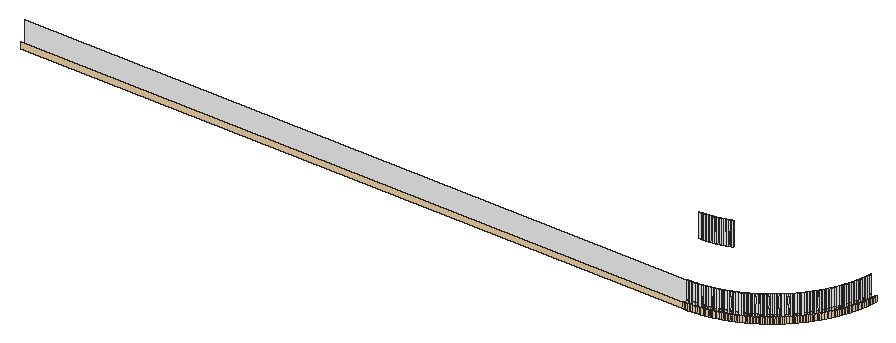
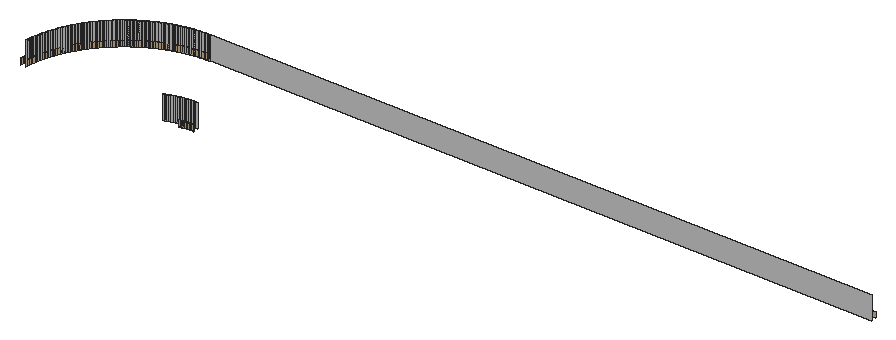
# SketchUp Ruby script. Lengths in inches.
U = 1.inch
M = Sketchup.active_model
def pt(a) = Geom::Point3d.new(a.map { |v| v * U })
def face(e, loops, mat)
  f = e.add_face(loops[0].map { |a| pt(a) })
  loops[1..].each { |l| e.add_face(l.map { |a| pt(a) }).erase! }
  f.material = f.back_material = mat if mat
  f
end
# faces: each face lists its corners as indices into pts; further lists are holes
def faces(e, pts, list, mat = nil) = list.each { |f| face(e, (f[0].is_a?(Array) ? f : [f]).map { |l| l.map { |i| pts[i] } }, mat) }
# xy, xz, yz: faces in a plane at the given z, y or x. An outline is a flat list of corners, or four numbers for a rectangle; further outlines are holes
def ring(l) = l.size == 4 ? [[l[0], l[1]], [l[2], l[1]], [l[2], l[3]], [l[0], l[3]]] : l.each_slice(2).to_a
def flat(e, list, mat, &to3) = list.each { |f| face(e, (f[0].is_a?(Array) ? f : [f]).map { |l| ring(l).map { |u, v| to3.(u, v) } }, mat) }
def xy(e, z, list, mat = nil) = flat(e, list, mat) { |x, y| [x, y, z] }
def xz(e, y, list, mat = nil) = flat(e, list, mat) { |x, z| [x, y, z] }
def yz(e, x, list, mat = nil) = flat(e, list, mat) { |y, z| [x, y, z] }
def lines(e, pts, list) = list.each { |a, b| e.add_line(pt(pts[a]), pt(pts[b])) }
# prism: a flat outline (further loops are holes) pulled along v
def prism(e, loops, v, mat = nil)
  f = face(e, loops, mat); d = Geom::Vector3d.new(v.map { |x| x * U })
  f.pushpull(f.normal.samedirection?(d) ? d.length : -d.length)
end
def box(e, o, s, mat = nil) = prism(e, [[o, [o[0] + s[0], o[1], o[2]], [o[0] + s[0], o[1] + s[1], o[2]], [o[0], o[1] + s[1], o[2]]]], [0, 0, s[2]], mat)
def at(x, y, z, deg = 0) = Geom::Transformation.translation(pt([x, y, z])) * Geom::Transformation.rotation(ORIGIN, Z_AXIS, deg.degrees)
def axes(o, x, y, z) = Geom::Transformation.new([*x, 0, *y, 0, *z, 0, *pt(o).to_a, 1])
def part(name) = M.definitions.add(name)
# library, detail: a bought-in or finely detailed component or shape, given as its bounding box
def library(name, o, s) = part(name).tap { |d| box(d.entities, o, s) }
def detail(e, o, s) = box(e.add_group.entities, o, s)
def put(e, d, t, mat = nil) = e.add_instance(d, t).tap { |i| i.material = mat if mat }
def group(e, t, mat = nil) = e.add_group.tap { |g| g.transformation = t; g.material = mat if mat }.entities
root = M.entities
M.materials.add("False Ceiling Light").color = [254, 223, 179]
M.materials.add("[Quartz Light Grey]").color = [251, 251, 252]
xz(root,43.5,[[45,115.32,177,116.49],[177,115.32,177.24,116.49],[177.24,115.32,177.47,116.49]],"False Ceiling Light")
xz(root,44.5,[[176.99,115.32,177.23,116.49],[177.23,115.32,177.45,116.49]],"False Ceiling Light")
xz(root,44.5,[[45.01,115.32,176.99,120],[176.99,115.32,177.23,120],[177.23,115.32,177.45,120]],"[Quartz Light Grey]")
xz(root,62.5,[[165.01,115.32,165.2,120]],"[Quartz Light Grey]")
xz(root,62.51,[[165.41,115.32,165.61,120]],"[Quartz Light Grey]")
xz(root,63.5,[[165.01,115.32,165.19,116.49],[165.19,115.32,165.38,116.49]],"False Ceiling Light")
p = [[177.47,43.5,115.32],[177.71,43.51,115.32],[177.71,43.51,116.49],[177.47,43.5,116.49],[177.94,43.52,115.32],[177.94,43.52,116.49],
  [178.18,43.53,115.32],[178.18,43.53,116.49],[178.41,43.54,115.32],[178.41,43.54,116.49],[178.65,43.56,115.32],[178.65,43.56,116.49],
  [178.88,43.58,115.32],[178.88,43.58,116.49],[179.12,43.6,115.32],[179.12,43.6,116.49],[179.35,43.625,115.32],[179.35,43.625,116.49],
  [179.59,43.65,115.32],[179.59,43.65,116.49],[179.82,43.68,115.32],[179.82,43.68,116.49],[180.05,43.71,115.32],[180.05,43.71,116.49],
  [180.29,43.74,115.32],[180.29,43.74,116.49],[180.52,43.78,115.32],[180.52,43.78,116.49],[180.75,43.82,115.32],[180.75,43.82,116.49],
  [180.98,43.86,115.32],[180.98,43.86,116.49],[181.22,43.9,115.32],[181.22,43.9,116.49],[181.45,43.94,115.32],[181.45,43.94,116.49],
  [181.68,43.99,115.32],[181.68,43.99,116.49],[181.91,44.04,115.32],[181.91,44.04,116.49],[182.14,44.09,115.32],[182.14,44.09,116.49],
  [182.37,44.15,115.32],[182.37,44.15,116.49],[182.6,44.21,115.32],[182.6,44.21,116.49],[182.82,44.27,115.32],[182.82,44.27,116.49],
  [183.05,44.33,115.32],[183.05,44.33,116.49],[183.28,44.39,115.32],[183.28,44.39,116.49],[183.5,44.46,115.32],[183.5,44.46,116.49],
  [177.45,44.5,115.32],[177.68,44.51,115.32],[177.68,44.51,120],[177.45,44.5,120],[177.68,44.51,115.32],[177.45,44.5,115.32],
  [177.45,44.5,116.49],[177.68,44.51,116.49],[177.9,44.52,115.32],[177.9,44.52,120],[177.9,44.52,115.32],[177.9,44.52,116.49],
  [178.125,44.53,115.32],[178.125,44.53,120],[178.125,44.53,115.32],[178.125,44.53,116.49],[178.35,44.54,115.32],[178.35,44.54,120],
  [178.35,44.54,115.32],[178.35,44.54,116.49],[178.57,44.56,115.32],[178.57,44.56,120],[178.57,44.56,115.32],[178.57,44.56,116.49],
  [183.73,44.53,115.32],[183.73,44.53,116.49],[183.95,44.6,115.32],[183.95,44.6,116.49],[178.8,44.58,115.32],[178.8,44.58,120],
  [178.8,44.58,115.32],[178.8,44.58,116.49],[179.02,44.6,115.32],[179.02,44.6,120],[179.02,44.6,115.32],[179.02,44.6,116.49],
  [179.25,44.62,115.32],[179.25,44.62,120],[179.25,44.62,115.32],[179.25,44.62,116.49],[179.47,44.64,115.32],[179.47,44.64,120],
  [179.47,44.64,115.32],[179.47,44.64,116.49],[179.69,44.67,115.32],[179.69,44.67,120],[179.69,44.67,115.32],[179.69,44.67,116.49],
  [184.18,44.68,115.32],[184.18,44.68,116.49],[179.92,44.7,115.32],[179.92,44.7,120],[179.92,44.7,115.32],[179.92,44.7,116.49],
  [180.14,44.73,115.32],[180.14,44.73,120],[180.14,44.73,115.32],[180.14,44.73,116.49],[180.36,44.76,115.32],[180.36,44.76,120],
  [180.36,44.76,115.32],[180.36,44.76,116.49],[184.4,44.75,115.32],[184.4,44.75,116.49],[180.59,44.8,115.32],[180.59,44.8,120],
  [180.59,44.8,115.32],[180.59,44.8,116.49],[180.81,44.84,115.32],[180.81,44.84,120],[180.81,44.84,115.32],[180.81,44.84,116.49],
  [181.03,44.88,115.32],[181.03,44.88,120],[181.03,44.88,115.32],[181.03,44.88,116.49],[184.62,44.83,115.32],[184.62,44.83,116.49],
  [184.84,44.91,115.32],[184.84,44.91,116.49],[181.25,44.92,115.32],[181.25,44.92,120],[181.25,44.92,115.32],[181.25,44.92,116.49],
  [181.47,44.97,115.32],[181.47,44.97,120],[181.47,44.97,115.32],[181.47,44.97,116.49],[185.0625,44.99,115.32],[185.0625,44.99,116.49],
  [181.69,45.02,115.32],[181.69,45.02,120],[181.69,45.02,115.32],[181.69,45.02,116.49],[181.91,45.07,115.32],[181.91,45.07,120],
  [181.91,45.07,115.32],[181.91,45.07,116.49],[185.28,45.08,115.32],[185.28,45.08,116.49],[182.13,45.12,115.32],[182.13,45.12,120],
  [182.13,45.12,115.32],[182.13,45.12,116.49],[182.35,45.18,115.32],[182.35,45.18,120],[182.35,45.18,115.32],[182.35,45.18,116.49],
  [185.5,45.17,115.32],[185.5,45.17,116.49],[182.56,45.23,115.32],[182.56,45.23,120],[182.56,45.23,115.32],[182.56,45.23,116.49],
  [182.78,45.29,115.32],[182.78,45.29,120],[182.78,45.29,115.32],[182.78,45.29,116.49],[185.72,45.26,115.32],[185.72,45.26,116.49],
  [183,45.35,115.32],[183,45.35,120],[183,45.35,115.32],[183,45.35,116.49],[185.9375,45.35,115.32],[185.9375,45.35,116.49],
  [183.21,45.42,115.32],[183.21,45.42,120],[183.21,45.42,115.32],[183.21,45.42,116.49],[183.43,45.48,115.32],[183.43,45.48,120],
  [183.43,45.48,115.32],[183.43,45.48,116.49],[186.15,45.45,115.32],[186.15,45.45,116.49],[186.37,45.54,115.32],[186.37,45.54,116.49],
  [183.64,45.55,115.32],[183.64,45.55,120],[183.64,45.55,115.32],[183.64,45.55,116.49],[186.58,45.64,115.32],[186.58,45.64,116.49],
  [183.86,45.625,115.32],[183.86,45.625,120],[183.86,45.625,115.32],[183.86,45.625,116.49],[184.07,45.7,115.32],[184.07,45.7,120],
  [184.07,45.7,115.32],[184.07,45.7,116.49],[186.79,45.74,115.32],[186.79,45.74,116.49],[184.28,45.77,115.32],[184.28,45.77,120],
  [184.28,45.77,115.32],[184.28,45.77,116.49],[187,45.85,115.32],[187,45.85,116.49],[184.49,45.85,115.32],[184.49,45.85,120],
  [184.49,45.85,115.32],[184.49,45.85,116.49],[184.7,45.93,115.32],[184.7,45.93,120],[184.7,45.93,115.32],[184.7,45.93,116.49],
  [187.21,45.95,115.32],[187.21,45.95,116.49],[184.91,46.01,115.32],[184.91,46.01,120],[184.91,46.01,115.32],[184.91,46.01,116.49],
  [185.125,46.09,115.32],[185.125,46.09,120],[185.125,46.09,115.32],[185.125,46.09,116.49],[187.42,46.06,115.32],[187.42,46.06,116.49],
  [185.33,46.18,115.32],[185.33,46.18,120],[185.33,46.18,115.32],[185.33,46.18,116.49],[187.63,46.17,115.32],[187.63,46.17,116.49],
  [185.54,46.27,115.32],[185.54,46.27,120],[185.54,46.27,115.32],[185.54,46.27,116.49],[187.84,46.28,115.32],[187.84,46.28,116.49],
  [185.74,46.36,115.32],[185.74,46.36,120],[185.74,46.36,115.32],[185.74,46.36,116.49],[188.05,46.4,115.32],[188.05,46.4,116.49],
  [185.95,46.45,115.32],[185.95,46.45,120],[185.95,46.45,115.32],[185.95,46.45,116.49],[188.25,46.51,115.32],[188.25,46.51,116.49],
  [186.15,46.55,115.32],[186.15,46.55,120],[186.15,46.55,115.32],[186.15,46.55,116.49],[186.36,46.64,115.32],[186.36,46.64,120],
  [186.36,46.64,115.32],[186.36,46.64,116.49],[188.45,46.63,115.32],[188.45,46.63,116.49],[186.56,46.74,115.32],[186.56,46.74,120],
  [186.56,46.74,115.32],[186.56,46.74,116.49],[188.66,46.75,115.32],[188.66,46.75,116.49],[186.76,46.84,115.32],[186.76,46.84,120],
  [186.76,46.84,115.32],[186.76,46.84,116.49],[186.96,46.95,115.32],[186.96,46.95,120],[186.96,46.95,115.32],[186.96,46.95,116.49],
  [188.86,46.88,115.32],[188.86,46.88,116.49],[187.16,47.05,115.32],[187.16,47.05,120],[187.16,47.05,115.32],[187.16,47.05,116.49],
  [189.06,47,115.32],[189.06,47,116.49],[189.25,47.13,115.32],[189.25,47.13,116.49],[187.36,47.16,115.32],[187.36,47.16,120],
  [187.36,47.16,115.32],[187.36,47.16,116.49],[189.45,47.26,115.32],[189.45,47.26,116.49],[187.55,47.27,115.32],[187.55,47.27,120],
  [187.55,47.27,115.32],[187.55,47.27,116.49],[187.75,47.38,115.32],[187.75,47.38,120],[187.75,47.38,115.32],[187.75,47.38,116.49],
  [189.65,47.39,115.32],[189.65,47.39,116.49],[187.94,47.49,115.32],[187.94,47.49,120],[187.94,47.49,115.32],[187.94,47.49,116.49],
  [189.84,47.52,115.32],[189.84,47.52,116.49],[188.14,47.61,115.32],[188.14,47.61,120],[188.14,47.61,115.32],[188.14,47.61,116.49],
  [190.03,47.66,115.32],[190.03,47.66,116.49],[188.33,47.73,115.32],[188.33,47.73,120],[188.33,47.73,115.32],[188.33,47.73,116.49],
  [188.52,47.85,115.32],[188.52,47.85,120],[188.52,47.85,115.32],[188.52,47.85,116.49],[190.23,47.8,115.32],[190.23,47.8,116.49],
  [188.71,47.97,115.32],[188.71,47.97,120],[188.71,47.97,115.32],[188.71,47.97,116.49],[190.42,47.9375,115.32],[190.42,47.9375,116.49],
  [190.6,48.08,115.32],[190.6,48.08,116.49],[188.9,48.09,115.32],[188.9,48.09,120],[188.9,48.09,115.32],[188.9,48.09,116.49],
  [189.08,48.22,115.32],[189.08,48.22,120],[189.08,48.22,115.32],[189.08,48.22,116.49],[190.79,48.22,115.32],[190.79,48.22,116.49],
  [189.27,48.35,115.32],[189.27,48.35,120],[189.27,48.35,115.32],[189.27,48.35,116.49],[190.98,48.37,115.32],[190.98,48.37,116.49],
  [189.45,48.47,115.32],[189.45,48.47,120],[189.45,48.47,115.32],[189.45,48.47,116.49],[191.16,48.51,115.32],[191.16,48.51,116.49],
  [189.64,48.61,115.32],[189.64,48.61,120],[189.64,48.61,115.32],[189.64,48.61,116.49],[191.34,48.66,115.32],[191.34,48.66,116.49],
  [189.82,48.74,115.32],[189.82,48.74,120],[189.82,48.74,115.32],[189.82,48.74,116.49],[190,48.875,115.32],[190,48.875,120],
  [190,48.875,115.32],[190,48.875,116.49],[191.52,48.81,115.32],[191.52,48.81,116.49],[191.7,48.97,115.32],[191.7,48.97,116.49],
  [190.18,49.01,115.32],[190.18,49.01,120],[190.18,49.01,115.32],[190.18,49.01,116.49],[190.35,49.15,115.32],[190.35,49.15,120],
  [190.35,49.15,115.32],[190.35,49.15,116.49],[191.88,49.12,115.32],[191.88,49.12,116.49],[192.06,49.28,115.32],[192.06,49.28,116.49],
  [190.53,49.29,115.32],[190.53,49.29,120],[190.53,49.29,115.32],[190.53,49.29,116.49],[190.7,49.43,115.32],[190.7,49.43,120],
  [190.7,49.43,115.32],[190.7,49.43,116.49],[192.23,49.4375,115.32],[192.23,49.4375,116.49],[190.88,49.58,115.32],[190.88,49.58,120],
  [190.88,49.58,115.32],[190.88,49.58,116.49],[192.4,49.6,115.32],[192.4,49.6,116.49],[191.05,49.72,115.32],[191.05,49.72,120],
  [191.05,49.72,115.32],[191.05,49.72,116.49],[192.57,49.76,115.32],[192.57,49.76,116.49],[191.22,49.87,115.32],[191.22,49.87,120],
  [191.22,49.87,115.32],[191.22,49.87,116.49],[192.74,49.92,115.32],[192.74,49.92,116.49],[191.39,50.02,115.32],[191.39,50.02,120],
  [191.39,50.02,115.32],[191.39,50.02,116.49],[192.91,50.09,115.32],[192.91,50.09,116.49],[191.55,50.17,115.32],[191.55,50.17,120],
  [191.55,50.17,115.32],[191.55,50.17,116.49],[193.08,50.26,115.32],[193.08,50.26,116.49],[191.72,50.33,115.32],[191.72,50.33,120],
  [191.72,50.33,115.32],[191.72,50.33,116.49],[191.88,50.48,115.32],[191.88,50.48,120],[191.88,50.48,115.32],[191.88,50.48,116.49],
  [193.24,50.43,115.32],[193.24,50.43,116.49],[193.4,50.6,115.32],[193.4,50.6,116.49],[192.04,50.64,115.32],[192.04,50.64,120],
  [192.04,50.64,115.32],[192.04,50.64,116.49],[192.2,50.8,115.32],[192.2,50.8,120],[192.2,50.8,115.32],[192.2,50.8,116.49],
  [193.5625,50.77,115.32],[193.5625,50.77,116.49],[192.36,50.96,115.32],[192.36,50.96,120],[192.36,50.96,115.32],[192.36,50.96,116.49],
  [193.72,50.94,115.32],[193.72,50.94,116.49],[193.88,51.12,115.32],[193.88,51.12,116.49],[192.52,51.12,115.32],[192.52,51.12,120],
  [192.52,51.12,115.32],[192.52,51.12,116.49],[192.67,51.28,115.32],[192.67,51.28,120],[192.67,51.28,115.32],[192.67,51.28,116.49],
  [194.03,51.3,115.32],[194.03,51.3,116.49],[192.83,51.45,115.32],[192.83,51.45,120],[192.83,51.45,115.32],[192.83,51.45,116.49],
  [194.19,51.48,115.32],[194.19,51.48,116.49],[192.98,51.61,115.32],[192.98,51.61,120],[192.98,51.61,115.32],[192.98,51.61,116.49],
  [194.34,51.66,115.32],[194.34,51.66,116.49],[193.13,51.78,115.32],[193.13,51.78,120],[193.13,51.78,115.32],[193.13,51.78,116.49],
  [194.49,51.84,115.32],[194.49,51.84,116.49],[193.28,51.95,115.32],[193.28,51.95,120],[193.28,51.95,115.32],[193.28,51.95,116.49],
  [194.63,52.02,115.32],[194.63,52.02,116.49],[193.42,52.12,115.32],[193.42,52.12,120],[193.42,52.12,115.32],[193.42,52.12,116.49],
  [194.78,52.21,115.32],[194.78,52.21,116.49],[193.57,52.3,115.32],[193.57,52.3,120],[193.57,52.3,115.32],[193.57,52.3,116.49],
  [194.92,52.4,115.32],[194.92,52.4,116.49],[193.71,52.47,115.32],[193.71,52.47,120],[193.71,52.47,115.32],[193.71,52.47,116.49],
  [195.0625,52.58,115.32],[195.0625,52.58,116.49],[193.85,52.65,115.32],[193.85,52.65,120],[193.85,52.65,115.32],[193.85,52.65,116.49],
  [193.99,52.82,115.32],[193.99,52.82,120],[193.99,52.82,115.32],[193.99,52.82,116.49],[195.2,52.77,115.32],[195.2,52.77,116.49],
  [194.125,53,115.32],[194.125,53,120],[194.125,53,115.32],[194.125,53,116.49],[195.34,52.97,115.32],[195.34,52.97,116.49],
  [194.26,53.18,115.32],[194.26,53.18,120],[194.26,53.18,115.32],[194.26,53.18,116.49],[195.48,53.16,115.32],[195.48,53.16,116.49],
  [194.39,53.36,115.32],[194.39,53.36,120],[194.39,53.36,115.32],[194.39,53.36,116.49],[195.61,53.35,115.32],[195.61,53.35,116.49],
  [194.53,53.55,115.32],[194.53,53.55,120],[194.53,53.55,115.32],[194.53,53.55,116.49],[195.74,53.55,115.32],[195.74,53.55,116.49],
  [194.65,53.73,115.32],[194.65,53.73,120],[194.65,53.73,115.32],[194.65,53.73,116.49],[195.87,53.75,115.32],[195.87,53.75,116.49],
  [194.78,53.92,115.32],[194.78,53.92,120],[194.78,53.92,115.32],[194.78,53.92,116.49],[196,53.94,115.32],[196,53.94,116.49],
  [194.91,54.1,115.32],[194.91,54.1,120],[194.91,54.1,115.32],[194.91,54.1,116.49],[196.12,54.14,115.32],[196.12,54.14,116.49],
  [195.03,54.29,115.32],[195.03,54.29,120],[195.03,54.29,115.32],[195.03,54.29,116.49],[196.25,54.34,115.32],[196.25,54.34,116.49],
  [195.15,54.48,115.32],[195.15,54.48,120],[195.15,54.48,115.32],[195.15,54.48,116.49],[196.37,54.55,115.32],[196.37,54.55,116.49],
  [195.27,54.67,115.32],[195.27,54.67,120],[195.27,54.67,115.32],[195.27,54.67,116.49],[196.49,54.75,115.32],[196.49,54.75,116.49],
  [195.39,54.86,115.32],[195.39,54.86,120],[195.39,54.86,115.32],[195.39,54.86,116.49],[196.6,54.95,115.32],[196.6,54.95,116.49],
  [195.51,55.06,115.32],[195.51,55.06,120],[195.51,55.06,115.32],[195.51,55.06,116.49],[196.72,55.16,115.32],[196.72,55.16,116.49],
  [195.62,55.25,115.32],[195.62,55.25,120],[195.62,55.25,115.32],[195.62,55.25,116.49],[196.83,55.37,115.32],[196.83,55.37,116.49],
  [195.73,55.45,115.32],[195.73,55.45,120],[195.73,55.45,115.32],[195.73,55.45,116.49],[195.84,55.64,115.32],[195.84,55.64,120],
  [195.84,55.64,115.32],[195.84,55.64,116.49],[196.94,55.58,115.32],[196.94,55.58,116.49],[195.95,55.84,115.32],[195.95,55.84,120],
  [195.95,55.84,115.32],[195.95,55.84,116.49],[197.05,55.79,115.32],[197.05,55.79,116.49],[196.05,56.04,115.32],[196.05,56.04,120],
  [196.05,56.04,115.32],[196.05,56.04,116.49],[197.15,56,115.32],[197.15,56,116.49],[196.16,56.24,115.32],[196.16,56.24,120],
  [196.16,56.24,115.32],[196.16,56.24,116.49],[197.26,56.21,115.32],[197.26,56.21,116.49],[196.26,56.44,115.32],[196.26,56.44,120],
  [196.26,56.44,115.32],[196.26,56.44,116.49],[197.36,56.42,115.32],[197.36,56.42,116.49],[196.36,56.64,115.32],[196.36,56.64,120],
  [196.36,56.64,115.32],[196.36,56.64,116.49],[197.46,56.63,115.32],[197.46,56.63,116.49],[196.45,56.85,115.32],[196.45,56.85,120],
  [196.45,56.85,115.32],[196.45,56.85,116.49],[197.55,56.85,115.32],[197.55,56.85,116.49],[196.55,57.05,115.32],[196.55,57.05,120],
  [196.55,57.05,115.32],[196.55,57.05,116.49],[197.65,57.0625,115.32],[197.65,57.0625,116.49],[196.64,57.26,115.32],[196.64,57.26,120],
  [196.64,57.26,115.32],[196.64,57.26,116.49],[197.74,57.28,115.32],[197.74,57.28,116.49],[196.73,57.46,115.32],[196.73,57.46,120],
  [196.73,57.46,115.32],[196.73,57.46,116.49],[197.83,57.5,115.32],[197.83,57.5,116.49],[196.82,57.67,115.32],[196.82,57.67,120],
  [196.82,57.67,115.32],[196.82,57.67,116.49],[197.92,57.72,115.32],[197.92,57.72,116.49],[196.91,57.875,115.32],[196.91,57.875,120],
  [196.91,57.875,115.32],[196.91,57.875,116.49],[198.01,57.9375,115.32],[198.01,57.9375,116.49],[196.99,58.09,115.32],[196.99,58.09,120],
  [196.99,58.09,115.32],[196.99,58.09,116.49],[198.09,58.16,115.32],[198.09,58.16,116.49],[197.07,58.3,115.32],[197.07,58.3,120],
  [197.07,58.3,115.32],[197.07,58.3,116.49],[198.17,58.38,115.32],[198.17,58.38,116.49],[197.15,58.51,115.32],[197.15,58.51,120],
  [197.15,58.51,115.32],[197.15,58.51,116.49],[198.25,58.6,115.32],[198.25,58.6,116.49],[197.23,58.72,115.32],[197.23,58.72,120],
  [197.23,58.72,115.32],[197.23,58.72,116.49],[198.32,58.82,115.32],[198.32,58.82,116.49],[197.3,58.93,115.32],[197.3,58.93,120],
  [197.3,58.93,115.32],[197.3,58.93,116.49],[198.4,59.05,115.32],[198.4,59.05,116.49],[197.375,59.14,115.32],[197.375,59.14,120],
  [197.375,59.14,115.32],[197.375,59.14,116.49],[198.47,59.27,115.32],[198.47,59.27,116.49],[197.45,59.36,115.32],[197.45,59.36,120],
  [197.45,59.36,115.32],[197.45,59.36,116.49],[198.54,59.5,115.32],[198.54,59.5,116.49],[197.52,59.57,115.32],[197.52,59.57,120],
  [197.52,59.57,115.32],[197.52,59.57,116.49],[198.61,59.72,115.32],[198.61,59.72,116.49],[197.58,59.79,115.32],[197.58,59.79,120],
  [197.58,59.79,115.32],[197.58,59.79,116.49],[198.67,59.95,115.32],[198.67,59.95,116.49],[197.65,60,115.32],[197.65,60,120],
  [197.65,60,115.32],[197.65,60,116.49],[198.73,60.18,115.32],[198.73,60.18,116.49],[197.71,60.22,115.32],[197.71,60.22,120],
  [197.71,60.22,115.32],[197.71,60.22,116.49],[197.77,60.44,115.32],[197.77,60.44,120],[197.77,60.44,115.32],[197.77,60.44,116.49],
  [198.79,60.4,115.32],[198.79,60.4,116.49],[197.82,60.65,115.32],[197.82,60.65,120],[197.82,60.65,115.32],[197.82,60.65,116.49],
  [198.85,60.63,115.32],[198.85,60.63,116.49],[198.91,60.86,115.32],[198.91,60.86,116.49],[197.88,60.87,115.32],[197.88,60.87,120],
  [197.88,60.87,115.32],[197.88,60.87,116.49],[197.93,61.09,115.32],[197.93,61.09,120],[197.93,61.09,115.32],[197.93,61.09,116.49],
  [198.96,61.09,115.32],[198.96,61.09,116.49],[197.98,61.31,115.32],[197.98,61.31,120],[197.98,61.31,115.32],[197.98,61.31,116.49],
  [199.01,61.32,115.32],[199.01,61.32,116.49],[198.03,61.53,115.32],[198.03,61.53,120],[198.03,61.53,115.32],[198.03,61.53,116.49],
  [199.06,61.55,115.32],[199.06,61.55,116.49],[198.08,61.75,115.32],[198.08,61.75,120],[198.08,61.75,115.32],[198.08,61.75,116.49],
  [199.1,61.78,115.32],[199.1,61.78,116.49],[198.12,61.97,115.32],[198.12,61.97,120],[198.12,61.97,115.32],[198.12,61.97,116.49],
  [199.14,62.02,115.32],[199.14,62.02,116.49],[198.16,62.19,115.32],[198.16,62.19,120],[198.16,62.19,115.32],[198.16,62.19,116.49],
  [199.18,62.25,115.32],[199.18,62.25,116.49],[198.2,62.41,115.32],[198.2,62.41,120],[198.2,62.41,115.32],[198.2,62.41,116.49],
  [199.22,62.48,115.32],[199.22,62.48,116.49],[198.24,62.64,115.32],[198.24,62.64,120],[198.24,62.64,115.32],[198.24,62.64,116.49],
  [165.41,62.51,115.32],[165.2,62.5,115.32],[165.2,62.5,120],[165.41,62.51,120],[165.8125,62.52,115.32],[165.61,62.51,115.32],
  [165.61,62.51,120],[165.8125,62.52,120],[166.01,62.53,115.32],[166.01,62.53,120],[166.22,62.55,115.32],[166.22,62.55,120],
  [166.42,62.56,115.32],[166.42,62.56,120],[199.26,62.71,115.32],[199.26,62.71,116.49],[166.62,62.58,115.32],[166.62,62.58,120],
  [166.82,62.61,115.32],[166.82,62.61,120],[167.02,62.63,115.32],[167.02,62.63,120],[167.22,62.66,115.32],[167.22,62.66,120],
  [198.27,62.86,115.32],[198.27,62.86,120],[198.27,62.86,115.32],[198.27,62.86,116.49],[167.42,62.69,115.32],[167.42,62.69,120],
  [167.625,62.72,115.32],[167.625,62.72,120],[167.82,62.76,115.32],[167.82,62.76,120],[199.29,62.95,115.32],[199.29,62.95,116.49],
  [168.02,62.8,115.32],[168.02,62.8,120],[168.22,62.84,115.32],[168.22,62.84,120],[168.42,62.88,115.32],[168.42,62.88,120],
  [168.62,62.93,115.32],[168.62,62.93,120],[168.82,62.98,115.32],[168.82,62.98,120],[198.3,63.08,115.32],[198.3,63.08,120],
  [198.3,63.08,115.32],[198.3,63.08,116.49],[199.32,63.18,115.32],[199.32,63.18,116.49],[169.01,63.03,115.32],[169.01,63.03,120],
  [169.21,63.08,115.32],[169.21,63.08,120],[169.4,63.14,115.32],[169.4,63.14,120],[169.6,63.2,115.32],[169.6,63.2,120],
  [198.33,63.31,115.32],[198.33,63.31,120],[198.33,63.31,115.32],[198.33,63.31,116.49],[169.79,63.26,115.32],[169.79,63.26,120],
  [199.35,63.41,115.32],[199.35,63.41,116.49],[169.98,63.32,115.32],[169.98,63.32,120],[170.17,63.39,115.32],[170.17,63.39,120],
  [198.36,63.53,115.32],[198.36,63.53,120],[198.36,63.53,115.32],[198.36,63.53,116.49],[170.36,63.46,115.32],[170.36,63.46,120],
  [199.375,63.65,115.32],[199.375,63.65,116.49],[165.38,63.5,115.32],[165.57,63.51,115.32],[165.57,63.51,116.49],[165.38,63.5,116.49],
  [165.76,63.52,115.32],[165.76,63.52,116.49],[165.95,63.53,115.32],[165.95,63.53,116.49],[166.14,63.54,115.32],[166.14,63.54,116.49],
  [166.33,63.5625,115.32],[166.33,63.5625,116.49],[170.55,63.53,115.32],[170.55,63.53,120],[170.74,63.6,115.32],[170.74,63.6,120],
  [198.38,63.75,115.32],[198.38,63.75,120],[198.38,63.75,115.32],[198.38,63.75,116.49],[166.52,63.58,115.32],[166.52,63.58,116.49],
  [166.7,63.6,115.32],[166.7,63.6,116.49],[166.89,63.625,115.32],[166.89,63.625,116.49],[167.08,63.65,115.32],[167.08,63.65,116.49],
  [170.93,63.68,115.32],[170.93,63.68,120],[199.4,63.88,115.32],[199.4,63.88,116.49],[167.27,63.68,115.32],[167.27,63.68,116.49],
  [167.46,63.71,115.32],[167.46,63.71,116.49],[167.64,63.74,115.32],[167.64,63.74,116.49],[167.83,63.78,115.32],[167.83,63.78,116.49],
  [171.12,63.76,115.32],[171.12,63.76,120]]
faces(root,p,[[0,1,2,3],[1,4,5,2],[4,6,7,5],[6,8,9,7],[8,10,11,9],[10,12,13,11],[12,14,15,13],[14,16,17,15],
  [16,18,19,17],[18,20,21,19],[20,22,23,21],[22,24,25,23],[24,26,27,25],[26,28,29,27],[28,30,31,29],[30,32,33,31],
  [32,34,35,33],[34,36,37,35],[36,38,39,37],[38,40,41,39],[40,42,43,41],[42,44,45,43],[44,46,47,45],[46,48,49,47],
  [48,50,51,49],[50,52,53,51],[58,59,60,61],[64,58,61,65],[68,64,65,69],[72,68,69,73],[76,72,73,77],[52,78,79,53],
  [78,80,81,79],[84,76,77,85],[88,84,85,89],[92,88,89,93],[96,92,93,97],[100,96,97,101],[80,102,103,81],[106,100,101,107],
  [110,106,107,111],[114,110,111,115],[102,116,117,103],[120,114,115,121],[124,120,121,125],[128,124,125,129],[116,130,131,117],[130,132,133,131],
  [136,128,129,137],[140,136,137,141],[132,142,143,133],[146,140,141,147],[150,146,147,151],[142,152,153,143],[156,150,151,157],[160,156,157,161],
  [152,162,163,153],[166,160,161,167],[170,166,167,171],[162,172,173,163],[176,170,171,177],[172,178,179,173],[182,176,177,183],[186,182,183,187],
  [178,188,189,179],[188,190,191,189],[194,186,187,195],[190,196,197,191],[200,194,195,201],[204,200,201,205],[196,206,207,197],[210,204,205,211],
  [206,212,213,207],[216,210,211,217],[220,216,217,221],[212,222,223,213],[226,220,221,227],[230,226,227,231],[222,232,233,223],[236,230,231,237],
  [232,238,239,233],[242,236,237,243],[238,244,245,239],[248,242,243,249],[244,250,251,245],[254,248,249,255],[250,256,257,251],[260,254,255,261],
  [264,260,261,265],[256,266,267,257],[270,264,265,271],[266,272,273,267],[276,270,271,277],[280,276,277,281],[272,282,283,273],[286,280,281,287],
  [282,288,289,283],[288,290,291,289],[294,286,287,295],[290,296,297,291],[300,294,295,301],[304,300,301,305],[296,306,307,297],[310,304,305,311],
  [306,312,313,307],[316,310,311,317],[312,318,319,313],[322,316,317,323],[326,322,323,327],[318,328,329,319],[332,326,327,333],[328,334,335,329],
  [334,336,337,335],[340,332,333,341],[344,340,341,345],[336,346,347,337],[350,344,345,351],[346,352,353,347],[356,350,351,357],[352,358,359,353],
  [362,356,357,363],[358,364,365,359],[368,362,363,369],[372,368,369,373],[364,374,375,365],[374,376,377,375],[380,372,373,381],[384,380,381,385],
  [376,386,387,377],[386,388,389,387],[392,384,385,393],[396,392,393,397],[388,398,399,389],[402,396,397,403],[398,404,405,399],[408,402,403,409],
  [404,410,411,405],[414,408,409,415],[410,416,417,411],[420,414,415,421],[416,422,423,417],[426,420,421,427],[422,428,429,423],[432,426,427,433],
  [436,432,433,437],[428,438,439,429],[438,440,441,439],[444,436,437,445],[448,444,445,449],[440,450,451,441],[454,448,449,455],[450,456,457,451],
  [456,458,459,457],[462,454,455,463],[466,462,463,467],[458,468,469,459],[472,466,467,473],[468,474,475,469],[478,472,473,479],[474,480,481,475],
  [484,478,479,485],[480,486,487,481],[490,484,485,491],[486,492,493,487],[496,490,491,497],[492,498,499,493],[502,496,497,503],[498,504,505,499],
  [508,502,503,509],[504,510,511,505],[514,508,509,515],[518,514,515,519],[510,520,521,511],[524,518,519,525],[520,526,527,521],[530,524,525,531],
  [526,532,533,527],[536,530,531,537],[532,538,539,533],[542,536,537,543],[538,544,545,539],[548,542,543,549],[544,550,551,545],[554,548,549,555],
  [550,556,557,551],[560,554,555,561],[556,562,563,557],[566,560,561,567],[562,568,569,563],[572,566,567,573],[568,574,575,569],[578,572,573,579],
  [574,580,581,575],[584,578,579,585],[580,586,587,581],[590,584,585,591],[586,592,593,587],[596,590,591,597],[592,598,599,593],[602,596,597,603],
  [606,602,603,607],[598,608,609,599],[612,606,607,613],[608,614,615,609],[618,612,613,619],[614,620,621,615],[624,618,619,625],[620,626,627,621],
  [630,624,625,631],[626,632,633,627],[636,630,631,637],[632,638,639,633],[642,636,637,643],[638,644,645,639],[648,642,643,649],[644,650,651,645],
  [654,648,649,655],[650,656,657,651],[660,654,655,661],[656,662,663,657],[666,660,661,667],[662,668,669,663],[672,666,667,673],[668,674,675,669],
  [678,672,673,679],[674,680,681,675],[684,678,679,685],[680,686,687,681],[690,684,685,691],[686,692,693,687],[696,690,691,697],[692,698,699,693],
  [702,696,697,703],[698,704,705,699],[708,702,703,709],[704,710,711,705],[714,708,709,715],[710,716,717,711],[720,714,715,721],[716,722,723,717],
  [726,720,721,727],[722,728,729,723],[732,726,727,733],[728,734,735,729],[738,732,733,739],[742,738,739,743],[734,744,745,735],[748,742,743,749],
  [744,750,751,745],[750,752,753,751],[756,748,749,757],[760,756,757,761],[752,762,763,753],[766,760,761,767],[762,768,769,763],[772,766,767,773],
  [768,774,775,769],[778,772,773,779],[774,780,781,775],[784,778,779,785],[780,786,787,781],[790,784,785,791],[786,792,793,787],[796,790,791,797],
  [792,798,799,793],[802,796,797,803],[798,818,819,799],[830,802,803,831],[818,838,839,819],[852,830,831,853],[838,854,855,839],[866,852,853,867],
  [854,870,871,855],[878,866,867,879],[870,882,883,871],[884,885,886,887],[885,888,889,886],[888,890,891,889],[890,892,893,891],[892,894,895,893],
  [902,878,879,903],[894,904,905,895],[904,906,907,905],[906,908,909,907],[908,910,911,909],[882,914,915,883],[910,916,917,911],[916,918,919,917],
  [918,920,921,919],[920,922,923,921]],"False Ceiling Light")
faces(root,p,[[54,55,56,57],[55,62,63,56],[62,66,67,63],[66,70,71,67],[70,74,75,71],[74,82,83,75],[82,86,87,83],[86,90,91,87],
  [90,94,95,91],[94,98,99,95],[98,104,105,99],[104,108,109,105],[108,112,113,109],[112,118,119,113],[118,122,123,119],[122,126,127,123],
  [126,134,135,127],[134,138,139,135],[138,144,145,139],[144,148,149,145],[148,154,155,149],[154,158,159,155],[158,164,165,159],[164,168,169,165],
  [168,174,175,169],[174,180,181,175],[180,184,185,181],[184,192,193,185],[192,198,199,193],[198,202,203,199],[202,208,209,203],[208,214,215,209],
  [214,218,219,215],[218,224,225,219],[224,228,229,225],[228,234,235,229],[234,240,241,235],[240,246,247,241],[246,252,253,247],[252,258,259,253],
  [258,262,263,259],[262,268,269,263],[268,274,275,269],[274,278,279,275],[278,284,285,279],[284,292,293,285],[292,298,299,293],[298,302,303,299],
  [302,308,309,303],[308,314,315,309],[314,320,321,315],[320,324,325,321],[324,330,331,325],[330,338,339,331],[338,342,343,339],[342,348,349,343],
  [348,354,355,349],[354,360,361,355],[360,366,367,361],[366,370,371,367],[370,378,379,371],[378,382,383,379],[382,390,391,383],[390,394,395,391],
  [394,400,401,395],[400,406,407,401],[406,412,413,407],[412,418,419,413],[418,424,425,419],[424,430,431,425],[430,434,435,431],[434,442,443,435],
  [442,446,447,443],[446,452,453,447],[452,460,461,453],[460,464,465,461],[464,470,471,465],[470,476,477,471],[476,482,483,477],[482,488,489,483],
  [488,494,495,489],[494,500,501,495],[500,506,507,501],[506,512,513,507],[512,516,517,513],[516,522,523,517],[522,528,529,523],[528,534,535,529],
  [534,540,541,535],[540,546,547,541],[546,552,553,547],[552,558,559,553],[558,564,565,559],[564,570,571,565],[570,576,577,571],[576,582,583,577],
  [582,588,589,583],[588,594,595,589],[594,600,601,595],[600,604,605,601],[604,610,611,605],[610,616,617,611],[616,622,623,617],[622,628,629,623],
  [628,634,635,629],[634,640,641,635],[640,646,647,641],[646,652,653,647],[652,658,659,653],[658,664,665,659],[664,670,671,665],[670,676,677,671],
  [676,682,683,677],[682,688,689,683],[688,694,695,689],[694,700,701,695],[700,706,707,701],[706,712,713,707],[712,718,719,713],[718,724,725,719],
  [724,730,731,725],[730,736,737,731],[736,740,741,737],[740,746,747,741],[746,754,755,747],[754,758,759,755],[758,764,765,759],[764,770,771,765],
  [770,776,777,771],[776,782,783,777],[782,788,789,783],[788,794,795,789],[794,800,801,795],[804,805,806,807],[808,809,810,811],[812,808,811,813],
  [814,812,813,815],[816,814,815,817],[820,816,817,821],[822,820,821,823],[824,822,823,825],[826,824,825,827],[800,828,829,801],[832,826,827,833],
  [834,832,833,835],[836,834,835,837],[840,836,837,841],[842,840,841,843],[844,842,843,845],[846,844,845,847],[848,846,847,849],[828,850,851,829],
  [856,848,849,857],[858,856,857,859],[860,858,859,861],[862,860,861,863],[850,864,865,851],[868,862,863,869],[872,868,869,873],[874,872,873,875],
  [864,876,877,865],[880,874,875,881],[896,880,881,897],[898,896,897,899],[876,900,901,877],[912,898,899,913],[924,912,913,925]],"[Quartz Light Grey]")
